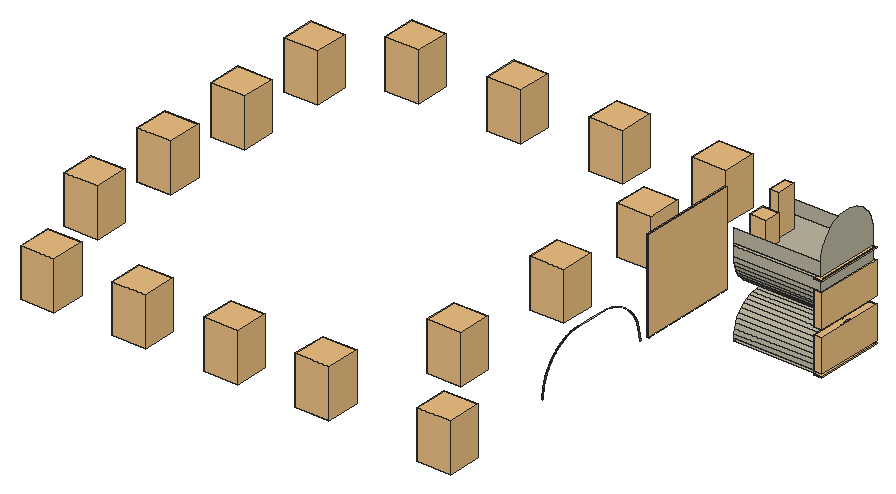
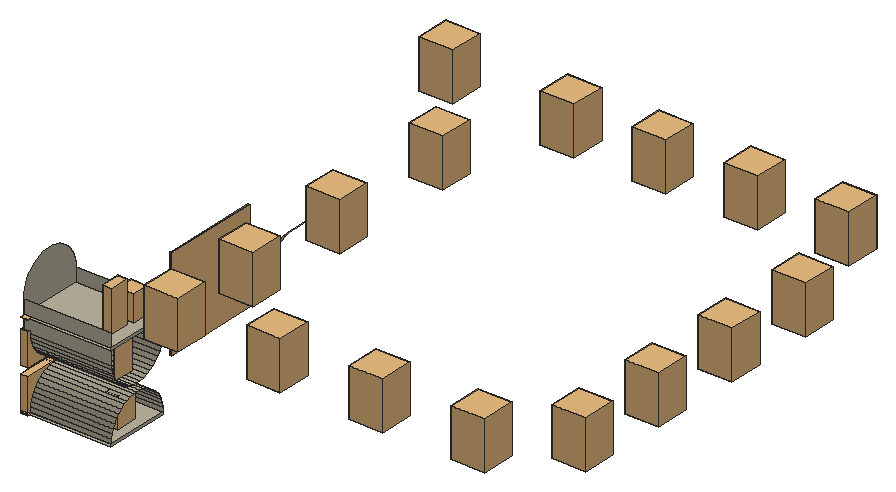
# SketchUp Ruby script. Lengths in inches.
U = 1.inch
M = Sketchup.active_model
def pt(a) = Geom::Point3d.new(a.map { |v| v * U })
def face(e, loops, mat)
  f = e.add_face(loops[0].map { |a| pt(a) })
  loops[1..].each { |l| e.add_face(l.map { |a| pt(a) }).erase! }
  f.material = f.back_material = mat if mat
  f
end
# faces: each face lists its corners as indices into pts; further lists are holes
def faces(e, pts, list, mat = nil) = list.each { |f| face(e, (f[0].is_a?(Array) ? f : [f]).map { |l| l.map { |i| pts[i] } }, mat) }
# xy, xz, yz: faces in a plane at the given z, y or x. An outline is a flat list of corners, or four numbers for a rectangle; further outlines are holes
def ring(l) = l.size == 4 ? [[l[0], l[1]], [l[2], l[1]], [l[2], l[3]], [l[0], l[3]]] : l.each_slice(2).to_a
def flat(e, list, mat, &to3) = list.each { |f| face(e, (f[0].is_a?(Array) ? f : [f]).map { |l| ring(l).map { |u, v| to3.(u, v) } }, mat) }
def xy(e, z, list, mat = nil) = flat(e, list, mat) { |x, y| [x, y, z] }
def xz(e, y, list, mat = nil) = flat(e, list, mat) { |x, z| [x, y, z] }
def yz(e, x, list, mat = nil) = flat(e, list, mat) { |y, z| [x, y, z] }
def lines(e, pts, list) = list.each { |a, b| e.add_line(pt(pts[a]), pt(pts[b])) }
# prism: a flat outline (further loops are holes) pulled along v
def prism(e, loops, v, mat = nil)
  f = face(e, loops, mat); d = Geom::Vector3d.new(v.map { |x| x * U })
  f.pushpull(f.normal.samedirection?(d) ? d.length : -d.length)
end
def box(e, o, s, mat = nil) = prism(e, [[o, [o[0] + s[0], o[1], o[2]], [o[0] + s[0], o[1] + s[1], o[2]], [o[0], o[1] + s[1], o[2]]]], [0, 0, s[2]], mat)
def at(x, y, z, deg = 0) = Geom::Transformation.translation(pt([x, y, z])) * Geom::Transformation.rotation(ORIGIN, Z_AXIS, deg.degrees)
def axes(o, x, y, z) = Geom::Transformation.new([*x, 0, *y, 0, *z, 0, *pt(o).to_a, 1])
def part(name) = M.definitions.add(name)
# library, detail: a bought-in or finely detailed component or shape, given as its bounding box
def library(name, o, s) = part(name).tap { |d| box(d.entities, o, s) }
def detail(e, o, s) = box(e.add_group.entities, o, s)
def put(e, d, t, mat = nil) = e.add_instance(d, t).tap { |i| i.material = mat if mat }
def group(e, t, mat = nil) = e.add_group.tap { |g| g.transformation = t; g.material = mat if mat }.entities
root = M.entities
M.materials.add("Tafisa-Terrarossa-PM780-4K").color = [148, 117, 107]
M.materials.add("Uniboard-L19-Putty-4K").color = [187, 181, 160]
c1 = library("Group\#20",[-0.5,-0.5,-0.1],[2,18,0.2])
c2 = library("Group\#25",[-0.5,-0.5,0],[2,18,8.5])
c3 = library("Alarm Clock 114 007",[-2.86,-1.17,0.01],[5.71,2.99,7.86])
c4 = library("Group\#27",[-0.5,-0.5,0],[2,18,8.5])
c5 = library("Picture 288 039",[-12.22,-0.48,-16.53],[24.44,0.48,33.06])
c6 = library("Group6\#1",[-12.88,-12,0],[25.76,24,0.5])
c7 = library("Group\#19",[-0.5,-0.5,-0.1],[2,18,0.2])
c8 = library("Decoration 111 063",[-2.51,-1.28,-0.03],[5.02,2.53,10.66])
c9 = library("Candle 111 040",[-2.11,-2.13,-0.02],[4.23,4.26,6.92])
c10 = library("Group\#17",[0,0,0],[8.9,8.9,12.62])
xy(root,80.79,[[120,120.5,141.83,137.5]],"Uniboard-L19-Putty-4K")
xy(root,81.5,[[120,120.5,142.83,137.5]],"Uniboard-L19-Putty-4K")
xy(root,93.88,[[119.96,92.62,120,118.38]],"Uniboard-L19-Putty-4K")
xy(root,103.27,[[120,120.5,141.83,137.5]],"Uniboard-L19-Putty-4K")
xy(root,103.98,[[120,120.5,142.83,137.5]],"Uniboard-L19-Putty-4K")
xy(root,106.125,[[119.29,70.41,119.53,70.6]],"Tafisa-Terrarossa-PM780-4K")
xy(root,106.125,[[119.29,70.6,119.53,74.5],[119.29,74.62,119.53,78.1875]],"Uniboard-L19-Putty-4K")
xz(root,58.62,[[119.29,94.14,119.53,94.33]],"Tafisa-Terrarossa-PM780-4K")
xz(root,92.62,[[119.96,94,120,118]],"Uniboard-L19-Putty-4K")
xz(root,118.38,[[119.96,94,120,118]],"Uniboard-L19-Putty-4K")
xz(root,120.5,[[120,100.5,142.83,103.27],[120,103.98,142.83,107.5]],"Uniboard-L19-Putty-4K")
xz(root,137.5,[[120,99.75,142.83,103.27],[120,103.98,142.83,107.5]],"Uniboard-L19-Putty-4K")
yz(root,119.96,[[92.62,94,118.38,118]],"Uniboard-L19-Putty-4K")
yz(root,120,[[120.5,80.79,137.5,81.5],[120.5,103.27,137.5,103.98]],"Uniboard-L19-Putty-4K")
yz(root,142.83,[[120.5,81.5,120.57,82.61,120.79,83.7,121.15,84.75,121.64,85.75,122.26,86.67,122.99,87.51,123.83,88.24,124.75,88.86,125.75,89.35,126.8,89.71,127.89,89.93,129,90,130.11,89.93,131.2,89.71,132.25,89.35,133.25,88.86,134.17,88.24,135.01,87.51,135.74,86.67,136.36,85.75,136.85,84.75,137.21,83.7,137.43,82.61,137.5,81.5],[129,92,127.89,92.07,126.8,92.29,125.75,92.65,124.75,93.14,123.83,93.76,122.99,94.49,122.26,95.33,121.64,96.25,121.15,97.25,120.79,98.3,120.57,99.39,120.5,100.5,120.5,103.27,137.5,103.27,137.5,99.75,137.34,98.71,137.05,97.7,136.64,96.73,136.12,95.82,135.48,94.98,134.75,94.23,133.93,93.57,133.04,93.02,132.08,92.58,131.08,92.26,130.05,92.06],[120.5,103.98,120.5,107.5,120.57,108.61,120.79,109.7,121.15,110.75,121.64,111.75,122.26,112.67,122.99,113.51,123.83,114.24,124.75,114.86,125.75,115.35,126.8,115.71,127.89,115.93,129,116,130.11,115.93,131.2,115.71,132.25,115.35,133.25,114.86,134.17,114.24,135.01,113.51,135.74,112.67,136.36,111.75,136.85,110.75,137.21,109.7,137.43,108.61,137.5,107.5,137.5,103.98]],"Uniboard-L19-Putty-4K")
p = [[120,120.57,82.61],[141.83,120.57,82.61],[141.83,120.5,81.5],[120,120.5,81.5],[120,137.5,81.5],[141.83,137.5,81.5],
  [141.83,137.43,82.61],[120,137.43,82.61],[120,120.79,83.7],[141.83,120.79,83.7],[141.83,137.21,83.7],[120,137.21,83.7],
  [120,121.15,84.75],[141.83,121.15,84.75],[141.83,136.85,84.75],[120,136.85,84.75],[120,121.64,85.75],[141.83,121.64,85.75],
  [141.83,136.36,85.75],[120,136.36,85.75],[120,122.26,86.67],[141.83,122.26,86.67],[141.83,135.74,86.67],[120,135.74,86.67],
  [120,122.99,87.51],[141.83,122.99,87.51],[141.83,135.01,87.51],[120,135.01,87.51],[120,123.83,88.24],[141.83,123.83,88.24],
  [141.83,134.17,88.24],[120,134.17,88.24],[120,124.75,88.86],[141.83,124.75,88.86],[141.83,133.25,88.86],[120,133.25,88.86],
  [120,125.75,89.35],[141.83,125.75,89.35],[141.83,132.25,89.35],[120,132.25,89.35],[120,126.8,89.71],[141.83,126.8,89.71],
  [141.83,131.2,89.71],[120,131.2,89.71],[120,127.89,89.93],[141.83,127.89,89.93],[141.83,130.11,89.93],[120,130.11,89.93],
  [120,129,90],[141.83,129,90],[120,127.89,92.07],[141.83,127.89,92.07],[141.83,129,92],[120,129,92],
  [141.83,130.05,92.06],[120,130.05,92.06],[120,126.8,92.29],[141.83,126.8,92.29],[141.83,131.08,92.26],[120,131.08,92.26],
  [120,125.75,92.65],[141.83,125.75,92.65],[141.83,132.08,92.58],[120,132.08,92.58],[120,124.75,93.14],[141.83,124.75,93.14],
  [141.83,133.04,93.02],[120,133.04,93.02],[141.83,133.93,93.57],[120,133.93,93.57],[120,123.83,93.76],[141.83,123.83,93.76],
  [141.83,134.75,94.23],[120,134.75,94.23],[119.29,90.39,95.42],[119.29,90.5,93.8125],[119.53,90.5,93.8125],[119.53,90.39,95.42],
  [120,122.99,94.49],[141.83,122.99,94.49],[141.83,135.48,94.98],[120,135.48,94.98],[119.29,58.62,94.33],[119.29,58.625,94.52],
  [119.53,58.625,94.52],[119.53,58.62,94.33],[119.29,58.63,94.71],[119.53,58.63,94.71],[120,122.26,95.33],[141.83,122.26,95.33],
  [119.29,58.64,94.9],[119.53,58.64,94.9],[119.29,58.66,95.08],[119.53,58.66,95.08],[141.83,136.12,95.82],[120,136.12,95.82],
  [119.29,58.67,95.27],[119.53,58.67,95.27],[119.29,58.69,95.46],[119.53,58.69,95.46],[120,121.64,96.25],[141.83,121.64,96.25],
  [119.29,90.08,97],[119.53,90.08,97],[119.29,58.71,95.64],[119.53,58.71,95.64],[119.29,58.74,95.83],[119.53,58.74,95.83],
  [119.29,58.77,96.02],[119.53,58.77,96.02],[141.83,136.64,96.73],[120,136.64,96.73],[119.29,58.8,96.2],[119.53,58.8,96.2],
  [119.29,58.83,96.39],[119.53,58.83,96.39],[120,121.15,97.25],[141.83,121.15,97.25],[119.29,58.87,96.57],[119.53,58.87,96.57],
  [119.29,58.91,96.76],[119.53,58.91,96.76],[141.83,137.05,97.7],[120,137.05,97.7],[119.29,58.95,96.94],[119.53,58.95,96.94],
  [119.29,58.99,97.12],[119.53,58.99,97.12],[119.29,89.5625,98.52],[119.53,89.5625,98.52],[119.29,59.04,97.3],[119.53,59.04,97.3],
  [120,120.79,98.3],[141.83,120.79,98.3],[119.29,59.09,97.49],[119.53,59.09,97.49],[119.29,59.15,97.67],[119.53,59.15,97.67],
  [119.29,59.2,97.85],[119.53,59.2,97.85],[141.83,137.34,98.71],[120,137.34,98.71],[119.29,59.26,98.02],[119.53,59.26,98.02],
  [119.29,59.33,98.2],[119.53,59.33,98.2],[119.29,59.39,98.38],[119.53,59.39,98.38],[120,120.57,99.39],[141.83,120.57,99.39],
  [119.29,59.46,98.55],[119.53,59.46,98.55],[119.29,88.85,99.97],[119.53,88.85,99.97],[119.29,59.53,98.73],[119.53,59.53,98.73],
  [119.29,59.6,98.9],[119.53,59.6,98.9],[141.83,137.5,99.75],[120,137.5,99.75],[119.29,59.68,99.07],[119.53,59.68,99.07],
  [119.29,22.22,99.06],[119.29,22.28,99.98],[119.53,22.28,99.98],[119.53,22.22,99.06],[119.29,36.3,99.98],[119.29,36.36,99.06],
  [119.53,36.36,99.06],[119.53,36.3,99.98],[119.29,59.76,99.24],[119.53,59.76,99.24],[119.29,59.84,99.41],[119.53,59.84,99.41],
  [119.29,59.92,99.58],[119.53,59.92,99.58],[120,120.5,100.5],[141.83,120.5,100.5],[119.29,60.01,99.75],[119.53,60.01,99.75],
  [119.29,60.1,99.92],[119.53,60.1,99.92],[119.29,60.19,100.08],[119.53,60.19,100.08],[119.29,22.46,100.89],[119.53,22.46,100.89],
  [119.29,36.12,100.89],[119.53,36.12,100.89],[119.29,87.96,101.31],[119.53,87.96,101.31],[119.29,60.29,100.24],[119.53,60.29,100.24],
  [119.29,60.38,100.4],[119.53,60.38,100.4],[119.29,60.48,100.5625],[119.53,60.48,100.5625],[119.29,60.59,100.72],[119.53,60.59,100.72],
  [119.29,60.69,100.88],[119.53,60.69,100.88],[119.29,22.76,101.76],[119.53,22.76,101.76],[119.29,35.82,101.76],[119.53,35.82,101.76],
  [119.29,60.8,101.03],[119.53,60.8,101.03],[119.29,60.91,101.1875],[119.53,60.91,101.1875],[119.29,61.02,101.34],[119.53,61.02,101.34],
  [119.29,61.13,101.49],[119.53,61.13,101.49],[119.29,86.89,102.52],[119.53,86.89,102.52],[119.29,61.25,101.63],[119.53,61.25,101.63],
  [119.29,61.37,101.78],[119.53,61.37,101.78],[119.29,23.17,102.59],[119.53,23.17,102.59],[119.29,35.41,102.59],[119.53,35.41,102.59],
  [119.29,61.49,101.92],[119.53,61.49,101.92],[119.29,61.61,102.07],[119.53,61.61,102.07],[119.29,61.74,102.21],[119.53,61.74,102.21],
  [119.29,61.87,102.35],[119.53,61.87,102.35],[119.29,62,102.48],[119.53,62,102.48],[119.29,62.13,102.62],[119.53,62.13,102.62],
  [119.29,85.68,103.58],[119.53,85.68,103.58],[119.29,23.68,103.36],[119.53,23.68,103.36],[119.29,34.9,103.36],[119.53,34.9,103.36],
  [119.29,62.26,102.75],[119.53,62.26,102.75],[119.29,62.4,102.88],[119.53,62.4,102.88],[119.29,62.54,103.01],[119.53,62.54,103.01],
  [119.29,62.68,103.13],[119.53,62.68,103.13],[119.29,62.82,103.25],[119.53,62.82,103.25],[119.29,62.96,103.375],[119.53,62.96,103.375],
  [119.29,24.29,104.05],[119.53,24.29,104.05],[119.29,34.29,104.05],[119.53,34.29,104.05],[119.29,63.11,103.49],[119.53,63.11,103.49],
  [119.29,63.26,103.61],[119.53,63.26,103.61],[119.29,63.41,103.72],[119.53,63.41,103.72],[119.29,84.34,104.48],[119.53,84.34,104.48],
  [119.29,63.56,103.84],[119.53,63.56,103.84],[119.29,63.71,103.95],[119.53,63.71,103.95],[119.29,63.87,104.05],[119.53,63.87,104.05],
  [119.29,24.99,104.66],[119.53,24.99,104.66],[119.29,33.6,104.66],[119.53,33.6,104.66],[119.29,64.02,104.16],[119.53,64.02,104.16],
  [119.29,64.18,104.26],[119.53,64.18,104.26],[119.29,64.34,104.36],[119.53,64.34,104.36],[119.29,64.5,104.46],[119.53,64.5,104.46],
  [119.29,64.66,104.55],[119.53,64.66,104.55],[119.29,82.9,105.1875],[119.53,82.9,105.1875],[119.29,64.83,104.64],[119.53,64.83,104.64],
  [119.29,64.99,104.73],[119.53,64.99,104.73],[119.29,25.76,105.18],[119.53,25.76,105.18],[119.29,32.83,105.18],[119.53,32.83,105.18],
  [119.29,65.16,104.82],[119.53,65.16,104.82],[119.29,65.33,104.9],[119.53,65.33,104.9],[119.29,65.5,104.98],[119.53,65.5,104.98],
  [119.29,65.67,105.0625],[119.53,65.67,105.0625],[119.29,65.84,105.14],[119.53,65.84,105.14],[119.29,66.01,105.21],[119.53,66.01,105.21],
  [119.29,26.59,105.59],[119.53,26.59,105.59],[119.29,32,105.59],[119.53,32,105.59],[119.29,66.1875,105.28],[119.53,66.1875,105.28],
  [119.29,81.375,105.71],[119.53,81.375,105.71],[119.29,66.36,105.35],[119.53,66.36,105.35],[119.29,66.54,105.42],[119.53,66.54,105.42],
  [119.29,66.72,105.48],[119.53,66.72,105.48],[119.29,66.9,105.54],[119.53,66.9,105.54],[119.29,67.08,105.6],[119.53,67.08,105.6],
  [119.29,27.46,105.88],[119.53,27.46,105.88],[119.29,31.12,105.88],[119.53,31.12,105.88],[119.29,67.26,105.65],[119.53,67.26,105.65],
  [119.29,67.4375,105.7],[119.53,67.4375,105.7],[119.29,67.62,105.75],[119.53,67.62,105.75],[119.29,67.8,105.79],[119.53,67.8,105.79],
  [119.29,79.79,106.02],[119.53,79.79,106.02],[119.29,67.99,105.84],[119.53,67.99,105.84],[119.29,68.17,105.875],[119.53,68.17,105.875],
  [119.29,28.37,106.06],[119.53,28.37,106.06],[119.29,30.22,106.06],[119.53,30.22,106.06],[119.29,68.35,105.91],[119.53,68.35,105.91],
  [119.29,68.54,105.95],[119.53,68.54,105.95],[119.29,68.73,105.98],[119.53,68.73,105.98],[119.29,68.91,106.01],[119.53,68.91,106.01],
  [119.29,69.1,106.03],[119.53,69.1,106.03],[119.29,69.29,106.05],[119.53,69.29,106.05],[119.29,78.1875,106.125],[119.53,78.1875,106.125],
  [119.29,29.29,106.125],[119.53,29.29,106.125],[119.29,69.47,106.07],[119.53,69.47,106.07],[119.29,69.66,106.09],[119.53,69.66,106.09],
  [119.29,69.85,106.1],[119.53,69.85,106.1],[119.29,70.04,106.11],[119.53,70.04,106.11],[119.29,70.22,106.12],[119.53,70.22,106.12],
  [119.29,70.41,106.125],[119.53,70.41,106.125]]
faces(root,p,[[0,1,2,3],[4,5,6,7],[8,9,1,0],[7,6,10,11],[12,13,9,8],[11,10,14,15],[16,17,13,12],[15,14,18,19],
  [20,21,17,16],[19,18,22,23],[24,25,21,20],[23,22,26,27],[28,29,25,24],[27,26,30,31],[32,33,29,28],[31,30,34,35],
  [36,37,33,32],[35,34,38,39],[40,41,37,36],[39,38,42,43],[44,45,41,40],[43,42,46,47],[48,49,45,44],[47,46,49,48],
  [50,51,52,53],[53,52,54,55],[56,57,51,50],[55,54,58,59],[60,61,57,56],[59,58,62,63],[64,65,61,60],[63,62,66,67],
  [67,66,68,69],[70,71,65,64],[69,68,72,73],[78,79,71,70],[73,72,80,81],[88,89,79,78],[81,80,94,95],[100,101,89,88],
  [95,94,110,111],[116,117,101,100],[111,110,122,123],[132,133,117,116],[123,122,140,141],[148,149,133,132],[141,140,158,159],[176,177,149,148]],"Uniboard-L19-Putty-4K")
faces(root,p,[[74,75,76,77],[82,83,84,85],[83,86,87,84],[86,90,91,87],[90,92,93,91],[92,96,97,93],[96,98,99,97],[102,74,77,103],
  [98,104,105,99],[104,106,107,105],[106,108,109,107],[108,112,113,109],[112,114,115,113],[114,118,119,115],[118,120,121,119],[120,124,125,121],
  [124,126,127,125],[128,102,103,129],[126,130,131,127],[130,134,135,131],[134,136,137,135],[136,138,139,137],[138,142,143,139],[142,144,145,143],
  [144,146,147,145],[146,150,151,147],[152,128,129,153],[150,154,155,151],[154,156,157,155],[156,160,161,157],[162,163,164,165],[166,167,168,169],
  [160,170,171,161],[170,172,173,171],[172,174,175,173],[174,178,179,175],[178,180,181,179],[180,182,183,181],[163,184,185,164],[186,166,169,187],
  [188,152,153,189],[182,190,191,183],[190,192,193,191],[192,194,195,193],[194,196,197,195],[196,198,199,197],[184,200,201,185],[202,186,187,203],
  [198,204,205,199],[204,206,207,205],[206,208,209,207],[208,210,211,209],[212,188,189,213],[210,214,215,211],[214,216,217,215],[200,218,219,201],
  [220,202,203,221],[216,222,223,217],[222,224,225,223],[224,226,227,225],[226,228,229,227],[228,230,231,229],[230,232,233,231],[234,212,213,235],
  [218,236,237,219],[238,220,221,239],[232,240,241,233],[240,242,243,241],[242,244,245,243],[244,246,247,245],[246,248,249,247],[248,250,251,249],
  [236,252,253,237],[254,238,239,255],[250,256,257,251],[256,258,259,257],[258,260,261,259],[262,234,235,263],[260,264,265,261],[264,266,267,265],
  [266,268,269,267],[252,270,271,253],[272,254,255,273],[268,274,275,269],[274,276,277,275],[276,278,279,277],[278,280,281,279],[280,282,283,281],
  [284,262,263,285],[282,286,287,283],[286,288,289,287],[270,290,291,271],[292,272,273,293],[288,294,295,289],[294,296,297,295],[296,298,299,297],
  [298,300,301,299],[300,302,303,301],[302,304,305,303],[290,306,307,291],[308,292,293,309],[304,310,311,305],[312,284,285,313],[310,314,315,311],
  [314,316,317,315],[316,318,319,317],[318,320,321,319],[320,322,323,321],[306,324,325,307],[326,308,309,327],[322,328,329,323],[328,330,331,329],
  [330,332,333,331],[332,334,335,333],[336,312,313,337],[334,338,339,335],[338,340,341,339],[324,342,343,325],[344,326,327,345],[340,346,347,341],
  [346,348,349,347],[348,350,351,349],[350,352,353,351],[352,354,355,353],[354,356,357,355],[358,336,337,359],[342,360,361,343],[360,344,345,361],
  [356,362,363,357],[362,364,365,363],[364,366,367,365],[366,368,369,367],[368,370,371,369],[370,372,373,371]],"Tafisa-Terrarossa-PM780-4K")
put(root,c1,at(141.83,120.5,80.79),"Uniboard-L19-Putty-4K")
put(root,c2,at(141.83,120.5,81.5),"Uniboard-L19-Putty-4K")
put(root,c3,at(123.72,129.23,81.5,-90))
put(root,c4,at(141.83,120.5,92),"Uniboard-L19-Putty-4K")
put(root,c5,axes([123.55,129.23,96.43],[0,-0.23328,0],[0.23328,0,0],[0,0,0.23328]))
put(root,c6,axes([119.96,105.5,106],[0,-1,0],[0,0,1],[-1,0,0]),"Uniboard-L19-Putty-4K")
put(root,c7,at(141.83,120.5,103.27),"Uniboard-L19-Putty-4K")
put(root,c8,at(124.81,130.23,103.98,-90))
put(root,c9,at(124.94,124.25,103.98,-90))
put(root,c10,at(22.18,9.19,105.17))
put(root,c10,at(46.18,9.19,105.17))
put(root,c10,at(70.18,9.19,105.17))
put(root,c10,at(94.18,9.19,105.17))
put(root,c10,at(127.74,7.07,105.17))
put(root,c10,at(106.59,123.42,105.38))
put(root,c10,at(106.59,98.88,105.38))
put(root,c10,at(106.59,70.57,105.38))
put(root,c10,at(106.59,36.76,105.38))
put(root,c10,at(79.78,123.42,105.38))
put(root,c10,at(52.97,123.42,105.38))
put(root,c10,at(26.16,123.42,105.38))
put(root,c10,at(10.36,110.22,105.38))
put(root,c10,at(10.36,86.22,105.38))
put(root,c10,at(10.36,62.22,105.38))
put(root,c10,at(10.36,38.22,105.38))
